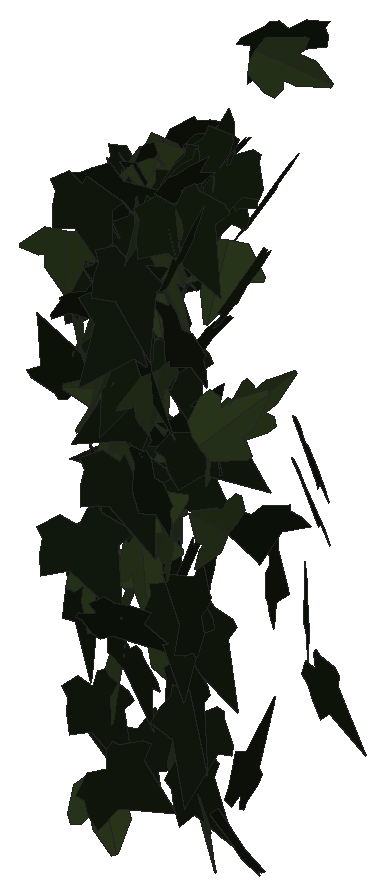
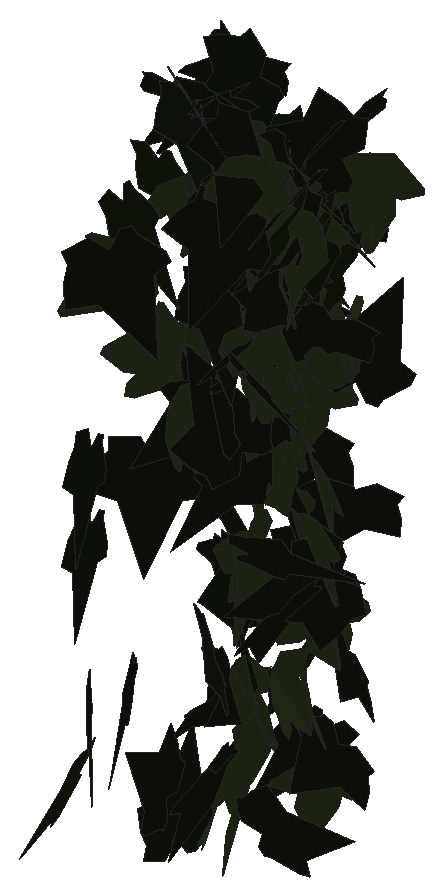
# SketchUp Ruby script. Lengths in inches.
U = 1.inch
M = Sketchup.active_model
def pt(a) = Geom::Point3d.new(a.map { |v| v * U })
def face(e, loops, mat)
  f = e.add_face(loops[0].map { |a| pt(a) })
  loops[1..].each { |l| e.add_face(l.map { |a| pt(a) }).erase! }
  f.material = f.back_material = mat if mat
  f
end
# faces: each face lists its corners as indices into pts; further lists are holes
def faces(e, pts, list, mat = nil) = list.each { |f| face(e, (f[0].is_a?(Array) ? f : [f]).map { |l| l.map { |i| pts[i] } }, mat) }
# xy, xz, yz: faces in a plane at the given z, y or x. An outline is a flat list of corners, or four numbers for a rectangle; further outlines are holes
def ring(l) = l.size == 4 ? [[l[0], l[1]], [l[2], l[1]], [l[2], l[3]], [l[0], l[3]]] : l.each_slice(2).to_a
def flat(e, list, mat, &to3) = list.each { |f| face(e, (f[0].is_a?(Array) ? f : [f]).map { |l| ring(l).map { |u, v| to3.(u, v) } }, mat) }
def xy(e, z, list, mat = nil) = flat(e, list, mat) { |x, y| [x, y, z] }
def xz(e, y, list, mat = nil) = flat(e, list, mat) { |x, z| [x, y, z] }
def yz(e, x, list, mat = nil) = flat(e, list, mat) { |y, z| [x, y, z] }
def lines(e, pts, list) = list.each { |a, b| e.add_line(pt(pts[a]), pt(pts[b])) }
# prism: a flat outline (further loops are holes) pulled along v
def prism(e, loops, v, mat = nil)
  f = face(e, loops, mat); d = Geom::Vector3d.new(v.map { |x| x * U })
  f.pushpull(f.normal.samedirection?(d) ? d.length : -d.length)
end
def box(e, o, s, mat = nil) = prism(e, [[o, [o[0] + s[0], o[1], o[2]], [o[0] + s[0], o[1] + s[1], o[2]], [o[0], o[1] + s[1], o[2]]]], [0, 0, s[2]], mat)
def at(x, y, z, deg = 0) = Geom::Transformation.translation(pt([x, y, z])) * Geom::Transformation.rotation(ORIGIN, Z_AXIS, deg.degrees)
def axes(o, x, y, z) = Geom::Transformation.new([*x, 0, *y, 0, *z, 0, *pt(o).to_a, 1])
def part(name) = M.definitions.add(name)
# library, detail: a bought-in or finely detailed component or shape, given as its bounding box
def library(name, o, s) = part(name).tap { |d| box(d.entities, o, s) }
def detail(e, o, s) = box(e.add_group.entities, o, s)
def put(e, d, t, mat = nil) = e.add_instance(d, t).tap { |i| i.material = mat if mat }
def group(e, t, mat = nil) = e.add_group.tap { |g| g.transformation = t; g.material = mat if mat }.entities
root = M.entities
M.materials.add("efeu1").color = [18, 25, 13]
M.materials.add("efeu2").color = [43, 57, 29]
c1 = part("ivyleaf_9")
p = [[1.54,2.16,1.25],[1.36,2.04,1.19],[-0.21,0.99,0.68],[-0.71,1.11,0.82],[-0.85,0.86,0.67],[-0.8,0.17,0.21],
  [-0.9,-0.01,0.1],[-0.67,-0.16,-0.02],[-0.08,-0.08,-0.05],[-0.03,-0.6,-0.4],[0.65,-0.88,-0.66],[0.83,-0.6,-0.49],
  [1.29,-0.42,-0.43],[1.8125,-0.07,-0.26],[1.21,0.44,0.15]]
faces(c1.entities,p,[[0,1,2,3,4,5,6,7,8,9,10,11,12,13,14]],"efeu1")
c2 = part("ivyleaf_10")
p = [[0,0.5,-0.03],[-0.0625,2.02,-0.43],[-0.19,2.01,-0.46],[-0.54,1.05,-0.29],[-0.52,0.625,-0.18],[-0.83,0.76,-0.28],
  [-1.16,0.64,-0.33],[-1.15,0.33,-0.24],[-0.77,-0.39,0.02],[-0.3,-0.51,0.16],[0.04,-0.48,0.23],[-0.02,2.01,-0.4375],
  [-0.06,2.01,-0.43],[0.04,-0.49,0.23],[0.67,-0.49,0.14],[1.38,0.36,-0.2],[1.375,0.51,-0.24],[0.81,0.65,-0.19],
  [0.62,0.59,-0.15],[0.6,1.09,-0.28],[0.5,1.23,-0.31]]
faces(c2.entities,p,[[0,1,2,3,4,5,6,7,8,9,10],[11,12,0,13,14,15,16,17,18,19,20]],"efeu2")
put(root,c1,axes([40.87,224.19,227.88],[-0.38704,0.07823,0.30673],[-0.31566,-0.0592,-0.38321],[-0.02364,-0.49028,0.09522]))
put(root,c1,axes([40.69,227.28,233.63],[0.01422,0.39948,-0.30035],[-0.10492,-0.29139,-0.39253],[-0.48866,0.07418,0.07554]))
put(root,c1,axes([40.6,222.42,229.75],[0.34458,-0.03291,0.36081],[-0.35457,0.07173,0.34516],[-0.07448,-0.49373,0.0261]))
put(root,c1,axes([40.34,222.9375,226.08],[-0.24159,-0.02636,-0.43697],[0.43663,0.02133,-0.24269],[0.03144,-0.49885,0.01271]))
put(root,c1,axes([40.26,223.4,231.1],[-0.06389,-0.30225,-0.39315],[0.27387,0.30896,-0.28203],[0.41342,-0.25138,0.12607]))
put(root,c2,axes([40.57,223.39,232],[-0.17407,0.40951,0.22805],[-0.09826,0.20598,-0.44488],[-0.45831,-0.19969,0.00876]))
put(root,c2,axes([40.47,222.93,230.22],[0.06282,-0.49564,-0.01975],[0.01702,-0.01774,0.4994],[-0.49575,-0.06342,0.01465]))
put(root,c2,axes([40.78,222.32,230.33],[0.0219,0.04263,-0.4977],[-0.22386,0.44619,0.02836],[0.44655,0.22159,0.03863]))
put(root,c2,axes([40.58,223.95,225.98],[0.16866,-0.39804,0.25123],[0.0892,-0.23501,-0.43222],[0.46217,0.19061,-0.00826]))
put(root,c2,axes([40.7,223.28,227.875],[0.41072,-0.23332,-0.16391],[-0.14317,0.07981,-0.47237],[0.24659,0.43496,-0.00125]))
put(root,c1,axes([40.43,223.125,227.18],[0.04917,0.19141,-0.45929],[0.02842,0.45969,0.19462],[0.49676,-0.04524,0.03432]))
put(root,c2,axes([40.59,223.23,228.78],[0.40654,-0.27018,0.1083],[0.08938,-0.06117,-0.48813],[0.27701,0.41625,-0.00144]))
put(root,c2,axes([40.78,221.97,232.43],[-0.41867,-0.27022,0.04112],[-0.03455,-0.0223,-0.49831],[0.27114,-0.4201,0]))
put(root,c1,axes([40.54,224.07,227.08],[0.0895,-0.48731,-0.06725],[-0.01354,0.06588,-0.49546],[0.49174,0.0905,-0.0014]))
put(root,c1,axes([40.48,223.33,232.16],[0.49242,-0.08494,-0.01744],[-0.01117,0.0376,-0.49846],[0.08599,0.4913,0.03513]))
put(root,c2,axes([40.7,222.92,226.53],[0.25936,0.41207,-0.11369],[-0.0634,-0.09443,-0.48689],[-0.42274,0.26698,0.00327]))
put(root,c2,axes([40.4,223.77,232.4],[-0.10038,-0.01704,-0.48952],[0.47616,0.11381,-0.1016],[0.11489,-0.48658,-0.00662]))
put(root,c1,axes([41.04,222.86,227.27],[0.02601,0.00613,0.49929],[-0.25022,0.43282,0.00772],[-0.43211,-0.25026,0.02558]))
put(root,c1,axes([40.49,224.01,232.65],[0.35939,-0.34423,0.04844],[0.03333,-0.03522,-0.49764],[0.34602,0.36093,-0.00237]))
put(root,c2,axes([40.89,223.34,232.29],[-0.39258,-0.30837,0.02811],[-0.01897,-0.02135,-0.49918],[0.30907,-0.393,0.00506]))
put(root,c1,axes([41,223.06,232.6],[-0.49327,0.05343,-0.06191],[0.05848,-0.03417,-0.49539],[-0.05717,-0.49596,0.02746]))
put(root,c1,axes([40.55,223.22,231.62],[0.26696,-0.42017,0.04678],[0.02039,-0.04247,-0.49778],[0.42228,0.26768,-0.00554]))
put(root,c1,axes([40.62,223.82,232.82],[0.11753,-0.4842,0.04163],[0.00172,-0.04242,-0.49819],[0.48599,0.11725,-0.00831]))
put(root,c1,axes([40.54,223.36,232.22],[0.39254,-0.30836,0.0287],[0.02082,-0.01995,-0.49917],[0.30899,0.39308,-0.00282]))
put(root,c2,axes([40.61,226.99,233.24],[0.24533,0.0565,0.43199],[0.2476,0.38985,-0.1916],[-0.35848,0.30794,0.16331]))
put(root,c1,axes([40.57,222.83,231.42],[0.35921,-0.31501,0.14743],[0.11151,-0.09645,-0.47777],[0.32945,0.37612,0.00097]))
put(root,c1,axes([40.83,222.95,232.21],[0.18972,-0.02395,-0.46199],[-0.18929,0.4516,-0.10114],[0.42211,0.21328,0.16229]))
put(root,c2,axes([40.97,223.76,232.87],[-0.17192,-0.45512,0.11537],[0.04401,-0.13794,-0.47858],[0.46745,-0.1544,0.08749]))
put(root,c2,axes([40.98,223.48,230.75],[0.1845,0.38465,-0.26078],[-0.13336,-0.22495,-0.42616],[-0.44517,0.22681,0.01959]))
put(root,c1,axes([40.71,222.7,224.51],[-0.16132,-0.10219,-0.4621],[0.40461,0.22347,-0.19067],[0.24549,-0.43545,0.01059]))
put(root,c2,axes([41,223.93,224.92],[-0.06726,0.21053,0.4485],[-0.11042,0.43486,-0.22069],[-0.48299,-0.12873,-0.012]))
put(root,c1,axes([40.57,223.75,232.46],[0.26053,-0.15527,0.39751],[0.34132,-0.20375,-0.30329],[0.25617,0.42939,-0.00017]))
put(root,c2,axes([41.29,222.86,229.68],[-0.04945,-0.02898,-0.4967],[-0.42144,-0.26288,0.0573],[-0.26447,0.42433,0.00157]))
put(root,c2,axes([41.04,223.97,233.17],[-0.34491,-0.33873,-0.12767],[0.08018,0.10048,-0.48319],[0.353,-0.35379,-0.015]))
put(root,c2,axes([40.73,223.75,231.61],[0.19031,-0.09904,0.45163],[0.39992,-0.20984,-0.21454],[0.23204,0.44289,-0.00065]))
put(root,c1,axes([41.4375,223.21,223.22],[-0.15153,0.07342,0.4708],[-0.42437,0.20385,-0.16838],[-0.21667,-0.45062,0.00054]))
put(root,c1,axes([40.89,222.22,233.26],[0.13691,-0.45794,-0.14678],[-0.03493,0.14274,-0.47792],[0.47962,0.14112,0.0071]))
put(root,c1,axes([41.27,223.2,231.95],[-0.49714,-0.02757,-0.0457],[0.04546,0.00574,-0.4979],[0.02797,-0.49921,-0.0032]))
put(root,c2,axes([41.36,223.76,225.66],[0.23918,-0.12181,-0.42185],[-0.32738,0.27064,-0.26377],[0.2926,0.40239,0.04971]))
put(root,c2,axes([41.15,222.64,229.59],[-0.17364,-0.44715,-0.14107],[0.06457,0.1262,-0.47948],[0.46441,-0.18474,0.01392]))
put(root,c1,axes([40.72,223.76,231.54],[0.23216,-0.09592,0.43232],[0.39556,-0.17454,-0.25114],[0.19909,0.45862,-0.00516]))
put(root,c1,axes([41.46,223.66,226.05],[-0.25443,0.21985,-0.37004],[-0.39759,0.04462,0.29988],[0.16488,0.44685,0.15212]))
put(root,c1,axes([41.13,224.28,232.61],[0.38661,0.3008,-0.10025],[-0.09314,-0.04337,-0.48933],[-0.30308,0.39704,0.02249]))
put(root,c1,axes([40.78,222.6,232.9375],[0.26291,-0.02751,0.4244],[0.42526,0.0233,-0.26193],[-0.00537,0.4987,0.03565]))
put(root,c2,axes([41.19,223.67,232.17],[-0.09468,0.30901,-0.38151],[-0.07201,-0.39308,-0.3005],[-0.48564,-0.00195,0.11894]))
put(root,c1,axes([41.07,224.73,224.82],[0.16107,-0.38446,-0.27613],[-0.1171,0.25024,-0.41673],[0.45863,0.19892,-0.00943]))
put(root,c1,axes([41.25,223.72,233.53],[0.16079,0.47134,0.04456],[0.02405,0.03887,-0.49791],[-0.47283,0.16226,-0.01017]))
put(root,c2,axes([41.03,222.88,225.16],[0.31871,-0.25291,0.29062],[0.22762,-0.18068,-0.40687],[0.31082,0.39165,-0.00004]))
put(root,c1,axes([41.48,223.73,230.17],[-0.48238,0.13153,0.00288],[-0.00302,-0.00012,-0.49999],[-0.13153,-0.48239,0.00091]))
put(root,c1,axes([41.3,221.8125,231.84],[0.17374,0.46881,-0.00578],[-0.00647,-0.00376,-0.49994],[-0.4688,0.1738,0.00476]))
put(root,c2,axes([41.24,222.72,229.59],[-0.02724,0.07319,-0.49386],[-0.07285,-0.48989,-0.06858],[-0.49391,0.06822,0.03735]))
put(root,c1,axes([41.06,221.92,227.7],[-0.13087,-0.27547,-0.39622],[0.1948,0.34543,-0.30451],[0.4415,-0.23408,0.01691]))
put(root,c2,axes([41.28,223.68,227.59],[0.04418,0.20405,-0.45433],[0.05042,0.45194,0.20788],[0.49549,-0.06418,0.01936]))
put(root,c2,axes([41.28,223.15,226.93],[0.09363,0.48906,-0.04529],[-0.00844,-0.0445,-0.49794],[-0.49108,0.09401,-0.00007]))
put(root,c2,axes([41.4,223.71,227.34],[0.11475,-0.41361,-0.25644],[-0.01798,0.25969,-0.42689],[0.48632,0.10719,0.04472]))
put(root,c2,axes([41.02,223.7,233.15],[0.26385,-0.01851,0.42431],[0.42102,0.07712,-0.25844],[-0.05588,0.49367,0.05628]))
put(root,c2,axes([41.53,223.28,230.27],[-0.41674,-0.25978,0.09405],[-0.07792,-0.05278,-0.49106],[0.26506,-0.42394,0.00351]))
put(root,c2,axes([41.13,223.09,230.1],[0.26564,-0.15251,0.39519],[0.35206,-0.17992,-0.30608],[0.23556,0.44087,0.01179]))
put(root,c1,axes([41.48,222.76,229.62],[-0.13383,-0.27804,0.39342],[-0.1943,-0.34249,-0.30814],[0.44084,-0.23536,-0.01638]))
put(root,c2,axes([41.54,222.61,232.74],[0.24197,-0.39207,-0.19424],[-0.04384,0.19911,-0.45654],[0.43535,0.23797,0.06198]))
put(root,c2,axes([41.36,222.34,230.65],[0.10599,-0.23425,0.42883],[0.21851,-0.36976,-0.25599],[0.43706,0.24167,0.02399]))
put(root,c2,axes([41.83,223.625,233.19],[-0.25414,-0.12611,0.41172],[-0.36686,-0.18689,-0.28369],[0.22545,-0.44628,0.00246]))
put(root,c1,axes([41.56,222.74,230.6],[-0.37349,-0.32676,-0.06115],[0.0492,0.03663,-0.49622],[0.32877,-0.37668,0.00479]))
put(root,c1,axes([41.39,222.48,228.64],[-0.19971,-0.2318,-0.39546],[0.24999,0.30649,-0.30589],[0.38422,-0.3199,-0.00652]))
put(root,c1,axes([41.31,222.8,225.33],[0.18328,-0.41186,0.21629],[0.10011,-0.1921,-0.45064],[0.4543,0.20849,0.01204]))
put(root,c1,axes([41.79,223.82,225.86],[0.00678,0.13941,0.48012],[-0.08221,0.47394,-0.13645],[-0.49315,-0.07709,0.02935]))
put(root,c2,axes([41.58,222.84,230.01],[-0.06685,0.47386,0.14487],[-0.03855,0.14077,-0.47822],[-0.49401,-0.07511,0.01772]))
put(root,c2,axes([41.9,222.4,228.58],[-0.31077,0.17254,-0.35164],[-0.30746,0.17066,0.35545],[0.24268,0.43716,0.00002]))
put(root,c2,axes([41.48,221.92,223.46],[0.31187,0.37841,0.09767],[0.06346,0.07426,-0.49036],[-0.38563,0.31826,-0.00171]))
put(root,c2,axes([41.68,222.74,227.8],[0.47154,0.10421,0.12958],[-0.12645,-0.0283,0.48292],[0.10799,-0.4882,-0.00034]))
put(root,c1,axes([41.71,223.16,231.59],[0.38104,0.09807,0.30853],[-0.30728,-0.04047,0.39236],[0.10193,-0.48861,0.02943]))
put(root,c1,axes([41.74,222.29,231.35],[-0.19813,-0.39588,0.23243],[-0.0787,-0.22011,-0.44199],[0.45227,-0.21173,0.02491]))
put(root,c1,axes([41.47,222.69,232.8],[0.46729,-0.17765,-0.00887],[-0.00726,0.00587,-0.49991],[0.17773,0.46734,0.0029]))
put(root,c1,axes([41.51,221.86,226.43],[0.45876,0.13092,0.14966],[0.1449,0.0376,-0.47706],[-0.13616,0.48109,-0.00345]))
put(root,c1,axes([41.59,223.44,230.31],[0.12871,-0.47248,-0.10099],[0.01288,0.10783,-0.48806],[0.48298,0.12304,0.03993]))
put(root,c1,axes([41.45,222.38,231.66],[0.04451,-0.06681,0.49351],[0.48105,-0.12245,-0.05996],[0.12888,0.48015,0.05338]))
put(root,c2,axes([41.96,223.05,223.49],[-0.17197,0.30608,0.35601],[-0.21206,0.28763,-0.34972],[-0.41888,-0.27127,0.03089]))
put(root,c1,axes([41.74,221.76,223.93],[0.07128,-0.11903,-0.48037],[-0.11017,0.46933,-0.13264],[0.48247,0.12475,0.04068]))
put(root,c1,axes([41.92,223.11,226.48],[0.05869,0.09856,0.48666],[0.08093,0.4816,-0.10729],[-0.4899,0.09136,0.04058]))
put(root,c1,axes([41.74,223.6,232.87],[-0.01731,-0.49956,-0.01195],[-0.00672,0.01219,-0.49981],[0.49966,-0.01714,-0.00714]))
put(root,c2,axes([41.95,223.18,231.41],[0.22714,-0.4194,-0.15003],[-0.05442,0.14102,-0.4766],[0.44209,0.23284,0.01841]))
put(root,c1,axes([41.76,223.26,228.43],[0.10668,-0.22287,-0.43468],[-0.08397,0.42994,-0.24105],[0.48122,0.12443,0.0543]))
put(root,c1,axes([41.6875,223.45,228.81],[0.33049,0.36569,0.08397],[-0.05756,-0.06117,0.4929],[0.37076,-0.33546,0.00167]))
put(root,c1,axes([42.12,225.09,226.05],[0.14434,-0.05005,-0.47609],[-0.42348,0.21852,-0.15137],[0.22322,0.44693,0.02069]))
put(root,c1,axes([42.34,223.55,233.53],[-0.19753,0.29118,0.35524],[-0.20381,0.29098,-0.35184],[-0.41163,-0.2838,0.00374]))
put(root,c2,axes([41.84,222.5,232.08],[0.42444,0.21073,0.15952],[0.13617,0.08429,-0.47366],[-0.22652,0.44552,0.01417]))
put(root,c1,axes([41.85,222.08,232.37],[0.09081,-0.48124,-0.10081],[-0.01326,0.10008,-0.4897],[0.49151,0.09161,0.00541]))
put(root,c1,axes([42.26,223.15,230.72],[-0.08595,0.49248,-0.00886],[0.01685,-0.00605,-0.49968],[-0.49227,-0.0862,-0.01555]))
put(root,c2,axes([42.24,222.48,227.83],[0.28208,-0.23885,-0.33673],[-0.17699,0.29848,-0.35998],[0.37297,0.32228,0.08384]))
put(root,c1,axes([42.34,222.05,228.9375],[0.16748,0.03564,-0.46977],[-0.46441,-0.07135,-0.17098],[-0.07922,0.4936,0.0092]))
put(root,c2,axes([42.17,222.3125,230.43],[-0.05582,-0.49633,-0.02336],[0.00255,0.02322,-0.49945],[0.49687,-0.05587,-0.00006]))
put(root,c2,axes([42.16,223.24,232.33],[-0.08973,-0.32729,-0.36719],[0.08346,0.35771,-0.33923],[0.48475,-0.12217,-0.00957]))
put(root,c1,axes([42.37,223.54,233.51],[-0.12411,0.48236,0.04393],[-0.00657,0.04366,-0.49805],[-0.48431,-0.1242,-0.0045]))
put(root,c1,axes([42.4,224.85,232.65],[-0.3053,0.36987,-0.14138],[0.07696,-0.11969,-0.47932],[-0.38842,-0.31444,0.01615]))
put(root,c1,axes([41.86,222.35,230.66],[0.04329,0.01081,-0.498],[0.4981,-0.006,0.04317],[-0.00504,-0.49985,-0.01129]))
put(root,c1,axes([41.94,223.59,228.83],[-0.0365,0.03246,0.49761],[0.27458,-0.41518,0.04722],[0.41626,0.27671,0.01248]))
put(root,c2,axes([42.05,222.5625,232.18],[-0.35734,0.15935,-0.31131],[0.25948,-0.1776,-0.38875],[-0.23447,-0.43939,0.04423]))
put(root,c1,axes([42.22,222.44,233.51],[0.21401,0.2989,0.3389],[0.14782,0.30805,-0.36504],[-0.42702,0.25644,0.04348]))
put(root,c2,axes([42.09,223.58,233.22],[0.3112,-0.17707,0.349],[0.3016,-0.17563,-0.35804],[0.24938,0.43336,-0.00251]))
put(root,c1,axes([42.16,223.02,225.08],[-0.19108,-0.02211,-0.46152],[0.45407,0.08343,-0.19199],[0.0855,-0.49249,-0.01181]))
put(root,c1,axes([42.34,223.6,233.45],[-0.19455,-0.4579,-0.04982],[0.01247,0.04883,-0.49745],[0.46043,-0.1948,-0.00758]))
put(root,c2,axes([42.34,223.83,229.17],[0.07988,-0.37587,0.31991],[0.14342,-0.29241,-0.37937],[0.47228,0.15237,0.0611]))
put(root,c1,axes([42.24,223.17,229.15],[-0.00618,-0.11646,-0.48621],[0.1243,0.47062,-0.1143],[0.48426,-0.12228,0.02313]))
put(root,c1,axes([42.34,222.67,226.58],[-0.31842,-0.13231,-0.36208],[0.33426,0.13919,-0.34481],[0.19204,-0.46165,-0.00019]))
put(root,c1,axes([42.71,225.2,225.61],[0.09115,-0.02363,-0.49105],[-0.47429,0.12721,-0.09416],[0.12939,0.48297,0.00077]))
put(root,c1,axes([42.41,223.52,233.29],[-0.11296,-0.45431,0.17563],[-0.00393,-0.17944,-0.46668],[0.48706,-0.10681,0.03697]))
put(root,c1,axes([42.61,223.58,233.77],[-0.42167,-0.23398,-0.1321],[0.14646,0.00594,-0.47803],[0.22527,-0.44184,0.06352]))
put(root,c2,axes([42.41,222.4,233.09],[-0.20907,0.23992,-0.38566],[0.22374,-0.31507,-0.31729],[-0.39526,-0.30524,0.02438]))
put(root,c1,axes([42.5,222.69,223.79],[0.2539,-0.31306,-0.29586],[-0.16722,0.24485,-0.4026],[0.39695,0.30338,0.01963]))
put(root,c2,axes([42.625,223.36,232.2],[0.25091,0.40407,-0.15419],[-0.08541,-0.12846,-0.47561],[-0.42397,0.26501,0.00456]))
put(root,c1,axes([42.86,222.08,231.6],[0.21604,0.08133,-0.44352],[-0.43789,-0.07954,-0.22788],[-0.10762,0.48689,0.03686]))
put(root,c1,axes([42.53,222.92,224.625],[-0.0567,-0.48926,0.0861],[-0.009,-0.08563,-0.49253],[0.49669,-0.0574,0.00091]))
put(root,c2,axes([42.58,222.86,223.19],[-0.2884,0.38042,-0.1487],[0.0901,-0.11829,-0.47738],[-0.39838,-0.30214,-0.00032]))
put(root,c1,axes([42.6,222.28,233.48],[-0.04818,-0.35679,-0.34696],[0.16586,0.31714,-0.34916],[0.46922,-0.14874,0.08779]))
put(root,c1,axes([42.97,224.85,227.78],[0.28051,0.03004,-0.41281],[-0.41157,0.07308,-0.27435],[0.04385,0.49372,0.06573]))
put(root,c1,axes([43.24,222,226.99],[-0.24542,0.05762,-0.4318],[-0.43403,0.01001,0.24802],[0.03722,0.49657,0.04511]))
put(root,c1,axes([43.11,221.67,233.02],[-0.0633,0.33083,0.36952],[-0.05459,0.3656,-0.33668],[-0.49296,-0.08297,-0.01016]))
put(root,c1,axes([42.93,223.39,223.32],[0.02994,-0.13882,0.47941],[0.18256,0.45004,0.11892],[-0.46452,0.16792,0.07763]))
put(root,c1,axes([42.86,225.28,224.43],[0.3562,-0.2992,-0.1833],[-0.13359,0.12589,-0.46509],[0.32447,0.3803,0.00974]))
put(root,c2,axes([42.97,223.4,229.63],[0.00995,-0.23744,0.43991],[0.00846,0.44002,0.23731],[-0.49983,0.00272,0.01278]))
put(root,c2,axes([43.07,222.8,228.01],[-0.084,-0.28864,-0.39954],[-0.0986,-0.38727,0.3005],[-0.48293,0.12928,0.00814]))
put(root,c1,axes([43.3125,223,232.125],[-0.24231,0.43245,0.06538],[-0.03712,0.05414,-0.49567],[-0.43579,-0.24507,0.00587]))
put(root,c1,axes([43.16,223.36,228.03],[0.23816,0.40634,-0.16783],[-0.10679,-0.13168,-0.47038],[-0.42647,0.25989,0.02407]))
put(root,c2,axes([42.84,222.82,229.53],[0.19947,0.17185,-0.42507],[0.32685,0.27178,0.26326],[0.32153,-0.38289,-0.00392]))
put(root,c1,axes([43.1875,224.59,228.7],[0.28683,0.00309,-0.40954],[-0.40672,0.06083,-0.28439],[0.04807,0.49628,0.03741]))
put(root,c1,axes([42.99,223.07,222.58],[0.44807,-0.22188,-0.00233],[0.0127,0.02039,0.49942],[-0.22153,-0.44761,0.02391]))
